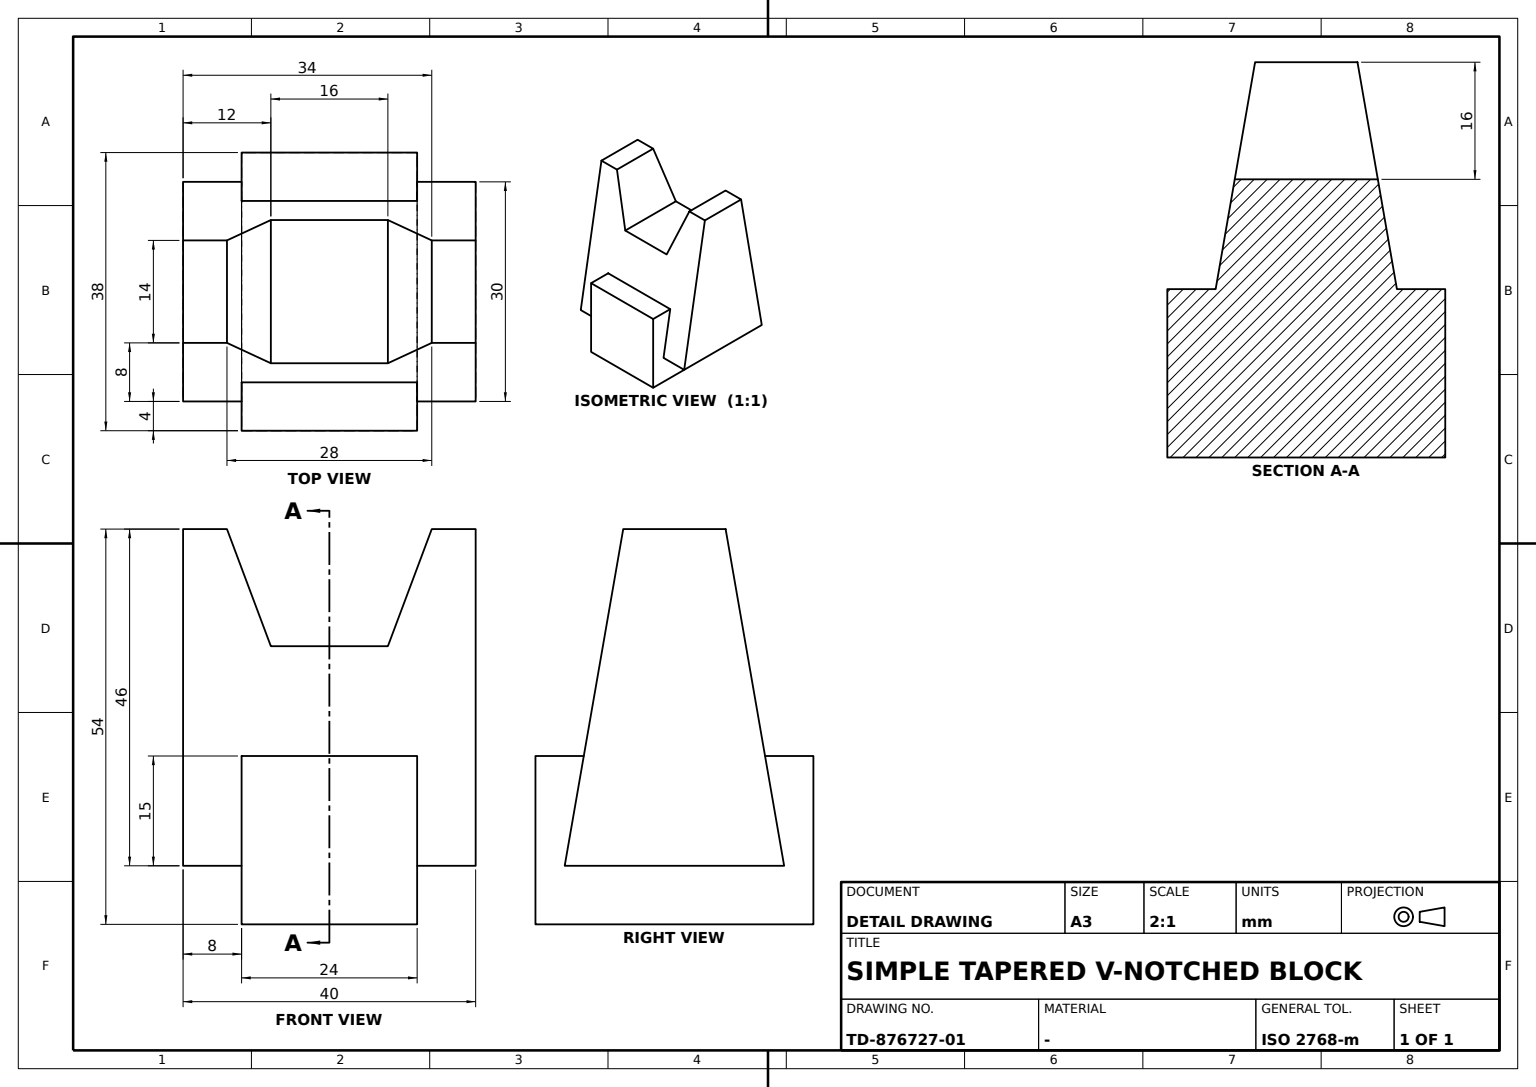
ISO-10303-21;
HEADER;
FILE_DESCRIPTION((''),'2;1');
FILE_NAME('','',(''),(''),'','','');
FILE_SCHEMA(('AUTOMOTIVE_DESIGN'));
ENDSEC;
DATA;
#1=APPLICATION_CONTEXT('');
#2=PRODUCT_CONTEXT('',#1,'mechanical');
#3=PRODUCT('','','',(#2));
#4=PRODUCT_DEFINITION_FORMATION('','',#3);
#5=PRODUCT_DEFINITION_CONTEXT('',#1,'design');
#6=PRODUCT_DEFINITION('','',#4,#5);
#7=PRODUCT_DEFINITION_SHAPE('','',#6);
#8=(LENGTH_UNIT()NAMED_UNIT(*)SI_UNIT(.MILLI.,.METRE.));
#9=(NAMED_UNIT(*)PLANE_ANGLE_UNIT()SI_UNIT($,.RADIAN.));
#10=(NAMED_UNIT(*)SI_UNIT($,.STERADIAN.)SOLID_ANGLE_UNIT());
#11=UNCERTAINTY_MEASURE_WITH_UNIT(LENGTH_MEASURE(0.005),#8,'distance_accuracy_value','');
#12=(GEOMETRIC_REPRESENTATION_CONTEXT(3)GLOBAL_UNCERTAINTY_ASSIGNED_CONTEXT((#11))GLOBAL_UNIT_ASSIGNED_CONTEXT((#8,#9,#10))REPRESENTATION_CONTEXT('',''));
#13=CARTESIAN_POINT('',(-7.,14.,46.));
#14=VERTEX_POINT('',#13);
#15=CARTESIAN_POINT('',(7.,14.,46.));
#16=VERTEX_POINT('',#15);
#17=CARTESIAN_POINT('',(0.,14.,46.));
#18=DIRECTION('',(1.,0.,0.));
#19=VECTOR('',#18,1000.);
#20=LINE('',#17,#19);
#21=EDGE_CURVE('',#14,#16,#20,.T.);
#22=ORIENTED_EDGE('',*,*,#21,.F.);
#23=CARTESIAN_POINT('',(-9.782609,8.,30.));
#24=VERTEX_POINT('',#23);
#25=CARTESIAN_POINT('',(-9.529906,8.54489,31.453041));
#26=DIRECTION('',(-0.160722869,-0.346558687,-0.924156499));
#27=VECTOR('',#26,1000.);
#28=LINE('',#25,#27);
#29=EDGE_CURVE('',#14,#24,#28,.T.);
#30=ORIENTED_EDGE('',*,*,#29,.T.);
#31=CARTESIAN_POINT('',(9.782609,8.,30.));
#32=VERTEX_POINT('',#31);
#33=CARTESIAN_POINT('',(0.,8.,30.));
#34=LINE('',#33,#19);
#35=EDGE_CURVE('',#24,#32,#34,.T.);
#36=ORIENTED_EDGE('',*,*,#35,.T.);
#37=CARTESIAN_POINT('',(9.529906,8.54489,31.453041));
#38=DIRECTION('',(0.160722869,-0.346558687,-0.924156499));
#39=VECTOR('',#38,1000.);
#40=LINE('',#37,#39);
#41=EDGE_CURVE('',#16,#32,#40,.T.);
#42=ORIENTED_EDGE('',*,*,#41,.F.);
#43=EDGE_LOOP('',(#22,#30,#36,#42));
#44=FACE_BOUND('',#43,.T.);
#45=DIRECTION('',(0.,0.936329178,-0.351123442));
#46=DIRECTION('',(0.,0.351123442,0.936329178));
#47=AXIS2_PLACEMENT_3D('',#33,#45,#46);
#48=PLANE('',#47);
#49=ADVANCED_FACE('',(#44),#48,.F.);
#50=CARTESIAN_POINT('',(-15.,-20.,0.));
#51=VERTEX_POINT('',#50);
#52=CARTESIAN_POINT('',(15.,-20.,0.));
#53=VERTEX_POINT('',#52);
#54=CARTESIAN_POINT('',(0.,-20.,0.));
#55=LINE('',#54,#19);
#56=EDGE_CURVE('',#51,#53,#55,.T.);
#57=ORIENTED_EDGE('',*,*,#56,.T.);
#58=CARTESIAN_POINT('',(7.,-20.,46.));
#59=VERTEX_POINT('',#58);
#60=DIRECTION('',(-0.171341175,0.,0.985211755));
#61=VECTOR('',#60,1000.);
#62=LINE('',#52,#61);
#63=EDGE_CURVE('',#53,#59,#62,.T.);
#64=ORIENTED_EDGE('',*,*,#63,.T.);
#65=CARTESIAN_POINT('',(-7.,-20.,46.));
#66=VERTEX_POINT('',#65);
#67=CARTESIAN_POINT('',(0.,-20.,46.));
#68=LINE('',#67,#19);
#69=EDGE_CURVE('',#66,#59,#68,.T.);
#70=ORIENTED_EDGE('',*,*,#69,.F.);
#71=DIRECTION('',(0.171341175,0.,0.985211755));
#72=VECTOR('',#71,1000.);
#73=LINE('',#50,#72);
#74=EDGE_CURVE('',#51,#66,#73,.T.);
#75=ORIENTED_EDGE('',*,*,#74,.F.);
#76=EDGE_LOOP('',(#57,#64,#70,#75));
#77=FACE_BOUND('',#76,.T.);
#78=DIRECTION('',(0.,1.,0.));
#79=DIRECTION('',(0.,0.,1.));
#80=AXIS2_PLACEMENT_3D('',#54,#78,#79);
#81=PLANE('',#80);
#82=ADVANCED_FACE('',(#77),#81,.F.);
#83=CARTESIAN_POINT('',(7.,-14.,46.));
#84=VERTEX_POINT('',#83);
#85=CARTESIAN_POINT('',(9.782609,-8.,30.));
#86=VERTEX_POINT('',#85);
#87=CARTESIAN_POINT('',(14.818975,2.859665,1.040892));
#88=DIRECTION('',(0.160722869,0.346558687,-0.924156499));
#89=VECTOR('',#88,1000.);
#90=LINE('',#87,#89);
#91=EDGE_CURVE('',#84,#86,#90,.T.);
#92=ORIENTED_EDGE('',*,*,#91,.T.);
#93=CARTESIAN_POINT('',(-9.782609,-8.,30.));
#94=VERTEX_POINT('',#93);
#95=CARTESIAN_POINT('',(0.,-8.,30.));
#96=LINE('',#95,#19);
#97=EDGE_CURVE('',#94,#86,#96,.T.);
#98=ORIENTED_EDGE('',*,*,#97,.F.);
#99=CARTESIAN_POINT('',(-7.,-14.,46.));
#100=VERTEX_POINT('',#99);
#101=CARTESIAN_POINT('',(-14.818975,2.859665,1.040892));
#102=DIRECTION('',(-0.160722869,0.346558687,-0.924156499));
#103=VECTOR('',#102,1000.);
#104=LINE('',#101,#103);
#105=EDGE_CURVE('',#100,#94,#104,.T.);
#106=ORIENTED_EDGE('',*,*,#105,.F.);
#107=CARTESIAN_POINT('',(0.,-14.,46.));
#108=LINE('',#107,#19);
#109=EDGE_CURVE('',#100,#84,#108,.T.);
#110=ORIENTED_EDGE('',*,*,#109,.T.);
#111=EDGE_LOOP('',(#92,#98,#106,#110));
#112=FACE_BOUND('',#111,.T.);
#113=DIRECTION('',(0.,-0.936329178,-0.351123442));
#114=DIRECTION('',(0.,0.351123442,-0.936329178));
#115=AXIS2_PLACEMENT_3D('',#107,#113,#114);
#116=PLANE('',#115);
#117=ADVANCED_FACE('',(#112),#116,.F.);
#118=CARTESIAN_POINT('',(19.,-12.,15.));
#119=VERTEX_POINT('',#118);
#120=CARTESIAN_POINT('',(19.,12.,15.));
#121=VERTEX_POINT('',#120);
#122=CARTESIAN_POINT('',(19.,0.,15.));
#123=VECTOR('',#78,1000.);
#124=LINE('',#122,#123);
#125=EDGE_CURVE('',#119,#121,#124,.T.);
#126=ORIENTED_EDGE('',*,*,#125,.F.);
#127=CARTESIAN_POINT('',(19.,-12.,-8.));
#128=VERTEX_POINT('',#127);
#129=CARTESIAN_POINT('',(19.,-12.,0.));
#130=DIRECTION('',(0.,0.,-1.));
#131=VECTOR('',#130,1000.);
#132=LINE('',#129,#131);
#133=EDGE_CURVE('',#119,#128,#132,.T.);
#134=ORIENTED_EDGE('',*,*,#133,.T.);
#135=CARTESIAN_POINT('',(19.,12.,-8.));
#136=VERTEX_POINT('',#135);
#137=CARTESIAN_POINT('',(19.,0.,-8.));
#138=DIRECTION('',(0.,-1.,0.));
#139=VECTOR('',#138,1000.);
#140=LINE('',#137,#139);
#141=EDGE_CURVE('',#136,#128,#140,.T.);
#142=ORIENTED_EDGE('',*,*,#141,.F.);
#143=VECTOR('',#79,1000.);
#144=LINE('',#120,#143);
#145=EDGE_CURVE('',#136,#121,#144,.T.);
#146=ORIENTED_EDGE('',*,*,#145,.T.);
#147=EDGE_LOOP('',(#126,#134,#142,#146));
#148=FACE_BOUND('',#147,.T.);
#149=CARTESIAN_POINT('',(19.,0.,0.));
#150=AXIS2_PLACEMENT_3D('',#149,#18,#78);
#151=PLANE('',#150);
#152=ADVANCED_FACE('',(#148),#151,.T.);
#153=CARTESIAN_POINT('',(-7.,20.,46.));
#154=VERTEX_POINT('',#153);
#155=LINE('',#13,#139);
#156=EDGE_CURVE('',#154,#14,#155,.T.);
#157=ORIENTED_EDGE('',*,*,#156,.F.);
#158=CARTESIAN_POINT('',(-15.,20.,0.));
#159=VERTEX_POINT('',#158);
#160=CARTESIAN_POINT('',(-6.794495,20.,47.181651));
#161=LINE('',#160,#72);
#162=EDGE_CURVE('',#159,#154,#161,.T.);
#163=ORIENTED_EDGE('',*,*,#162,.F.);
#164=CARTESIAN_POINT('',(-15.,12.,0.));
#165=VERTEX_POINT('',#164);
#166=CARTESIAN_POINT('',(-15.,0.,0.));
#167=LINE('',#166,#139);
#168=EDGE_CURVE('',#159,#165,#167,.T.);
#169=ORIENTED_EDGE('',*,*,#168,.T.);
#170=CARTESIAN_POINT('',(-12.391304,12.,15.));
#171=VERTEX_POINT('',#170);
#172=CARTESIAN_POINT('',(-12.027523,12.,17.091743));
#173=LINE('',#172,#72);
#174=EDGE_CURVE('',#165,#171,#173,.T.);
#175=ORIENTED_EDGE('',*,*,#174,.T.);
#176=CARTESIAN_POINT('',(-12.391304,-12.,15.));
#177=VERTEX_POINT('',#176);
#178=CARTESIAN_POINT('',(-12.391304,0.,15.));
#179=LINE('',#178,#123);
#180=EDGE_CURVE('',#177,#171,#179,.T.);
#181=ORIENTED_EDGE('',*,*,#180,.F.);
#182=CARTESIAN_POINT('',(-15.,-12.,0.));
#183=VERTEX_POINT('',#182);
#184=CARTESIAN_POINT('',(-12.027523,-12.,17.091743));
#185=LINE('',#184,#72);
#186=EDGE_CURVE('',#183,#177,#185,.T.);
#187=ORIENTED_EDGE('',*,*,#186,.F.);
#188=EDGE_CURVE('',#183,#51,#167,.T.);
#189=ORIENTED_EDGE('',*,*,#188,.T.);
#190=ORIENTED_EDGE('',*,*,#74,.T.);
#191=EDGE_CURVE('',#100,#66,#155,.T.);
#192=ORIENTED_EDGE('',*,*,#191,.F.);
#193=ORIENTED_EDGE('',*,*,#105,.T.);
#194=CARTESIAN_POINT('',(-9.782609,0.,30.));
#195=LINE('',#194,#123);
#196=EDGE_CURVE('',#94,#24,#195,.T.);
#197=ORIENTED_EDGE('',*,*,#196,.T.);
#198=ORIENTED_EDGE('',*,*,#29,.F.);
#199=EDGE_LOOP('',(#157,#163,#169,#175,#181,#187,#189,#190,#192,#193,#197,#198));
#200=FACE_BOUND('',#199,.T.);
#201=DIRECTION('',(0.985211755,0.,-0.171341175));
#202=AXIS2_PLACEMENT_3D('',#166,#201,#71);
#203=PLANE('',#202);
#204=ADVANCED_FACE('',(#200),#203,.F.);
#205=CARTESIAN_POINT('',(7.,20.,46.));
#206=VERTEX_POINT('',#205);
#207=CARTESIAN_POINT('',(0.,20.,46.));
#208=LINE('',#207,#19);
#209=EDGE_CURVE('',#154,#206,#208,.T.);
#210=ORIENTED_EDGE('',*,*,#209,.T.);
#211=CARTESIAN_POINT('',(15.,20.,0.));
#212=VERTEX_POINT('',#211);
#213=CARTESIAN_POINT('',(6.794495,20.,47.181651));
#214=LINE('',#213,#61);
#215=EDGE_CURVE('',#212,#206,#214,.T.);
#216=ORIENTED_EDGE('',*,*,#215,.F.);
#217=CARTESIAN_POINT('',(0.,20.,0.));
#218=LINE('',#217,#19);
#219=EDGE_CURVE('',#159,#212,#218,.T.);
#220=ORIENTED_EDGE('',*,*,#219,.F.);
#221=ORIENTED_EDGE('',*,*,#162,.T.);
#222=EDGE_LOOP('',(#210,#216,#220,#221));
#223=FACE_BOUND('',#222,.T.);
#224=AXIS2_PLACEMENT_3D('',#207,#138,#130);
#225=PLANE('',#224);
#226=ADVANCED_FACE('',(#223),#225,.F.);
#227=CARTESIAN_POINT('',(-19.,-12.,-8.));
#228=VERTEX_POINT('',#227);
#229=CARTESIAN_POINT('',(0.,-12.,-8.));
#230=LINE('',#229,#19);
#231=EDGE_CURVE('',#228,#128,#230,.T.);
#232=ORIENTED_EDGE('',*,*,#231,.T.);
#233=ORIENTED_EDGE('',*,*,#133,.F.);
#234=CARTESIAN_POINT('',(12.391304,-12.,15.));
#235=VERTEX_POINT('',#234);
#236=CARTESIAN_POINT('',(0.,-12.,15.));
#237=LINE('',#236,#19);
#238=EDGE_CURVE('',#235,#119,#237,.T.);
#239=ORIENTED_EDGE('',*,*,#238,.F.);
#240=CARTESIAN_POINT('',(15.,-12.,0.));
#241=VERTEX_POINT('',#240);
#242=CARTESIAN_POINT('',(12.027523,-12.,17.091743));
#243=LINE('',#242,#61);
#244=EDGE_CURVE('',#241,#235,#243,.T.);
#245=ORIENTED_EDGE('',*,*,#244,.F.);
#246=CARTESIAN_POINT('',(0.,-12.,0.));
#247=LINE('',#246,#19);
#248=EDGE_CURVE('',#183,#241,#247,.T.);
#249=ORIENTED_EDGE('',*,*,#248,.F.);
#250=ORIENTED_EDGE('',*,*,#186,.T.);
#251=CARTESIAN_POINT('',(-19.,-12.,15.));
#252=VERTEX_POINT('',#251);
#253=EDGE_CURVE('',#252,#177,#237,.T.);
#254=ORIENTED_EDGE('',*,*,#253,.F.);
#255=CARTESIAN_POINT('',(-19.,-12.,0.));
#256=LINE('',#255,#131);
#257=EDGE_CURVE('',#252,#228,#256,.T.);
#258=ORIENTED_EDGE('',*,*,#257,.T.);
#259=EDGE_LOOP('',(#232,#233,#239,#245,#249,#250,#254,#258));
#260=FACE_BOUND('',#259,.T.);
#261=AXIS2_PLACEMENT_3D('',#236,#138,#130);
#262=PLANE('',#261);
#263=ADVANCED_FACE('',(#260),#262,.T.);
#264=CARTESIAN_POINT('',(9.782609,0.,30.));
#265=LINE('',#264,#123);
#266=EDGE_CURVE('',#86,#32,#265,.T.);
#267=ORIENTED_EDGE('',*,*,#266,.T.);
#268=ORIENTED_EDGE('',*,*,#35,.F.);
#269=ORIENTED_EDGE('',*,*,#196,.F.);
#270=ORIENTED_EDGE('',*,*,#97,.T.);
#271=EDGE_LOOP('',(#267,#268,#269,#270));
#272=FACE_BOUND('',#271,.T.);
#273=AXIS2_PLACEMENT_3D('',#95,#130,#78);
#274=PLANE('',#273);
#275=ADVANCED_FACE('',(#272),#274,.F.);
#276=ORIENTED_EDGE('',*,*,#191,.T.);
#277=ORIENTED_EDGE('',*,*,#69,.T.);
#278=LINE('',#15,#139);
#279=EDGE_CURVE('',#84,#59,#278,.T.);
#280=ORIENTED_EDGE('',*,*,#279,.F.);
#281=ORIENTED_EDGE('',*,*,#109,.F.);
#282=EDGE_LOOP('',(#276,#277,#280,#281));
#283=FACE_BOUND('',#282,.T.);
#284=AXIS2_PLACEMENT_3D('',#17,#130,#78);
#285=PLANE('',#284);
#286=ADVANCED_FACE('',(#283),#285,.F.);
#287=ORIENTED_EDGE('',*,*,#141,.T.);
#288=ORIENTED_EDGE('',*,*,#231,.F.);
#289=CARTESIAN_POINT('',(-19.,12.,-8.));
#290=VERTEX_POINT('',#289);
#291=CARTESIAN_POINT('',(-19.,0.,-8.));
#292=LINE('',#291,#139);
#293=EDGE_CURVE('',#290,#228,#292,.T.);
#294=ORIENTED_EDGE('',*,*,#293,.F.);
#295=CARTESIAN_POINT('',(0.,12.,-8.));
#296=LINE('',#295,#19);
#297=EDGE_CURVE('',#290,#136,#296,.T.);
#298=ORIENTED_EDGE('',*,*,#297,.T.);
#299=EDGE_LOOP('',(#287,#288,#294,#298));
#300=FACE_BOUND('',#299,.T.);
#301=AXIS2_PLACEMENT_3D('',#295,#79,#138);
#302=PLANE('',#301);
#303=ADVANCED_FACE('',(#300),#302,.F.);
#304=CARTESIAN_POINT('',(15.,12.,0.));
#305=VERTEX_POINT('',#304);
#306=CARTESIAN_POINT('',(15.,0.,0.));
#307=LINE('',#306,#139);
#308=EDGE_CURVE('',#212,#305,#307,.T.);
#309=ORIENTED_EDGE('',*,*,#308,.F.);
#310=ORIENTED_EDGE('',*,*,#215,.T.);
#311=EDGE_CURVE('',#206,#16,#278,.T.);
#312=ORIENTED_EDGE('',*,*,#311,.T.);
#313=ORIENTED_EDGE('',*,*,#41,.T.);
#314=ORIENTED_EDGE('',*,*,#266,.F.);
#315=ORIENTED_EDGE('',*,*,#91,.F.);
#316=ORIENTED_EDGE('',*,*,#279,.T.);
#317=ORIENTED_EDGE('',*,*,#63,.F.);
#318=EDGE_CURVE('',#241,#53,#307,.T.);
#319=ORIENTED_EDGE('',*,*,#318,.F.);
#320=ORIENTED_EDGE('',*,*,#244,.T.);
#321=CARTESIAN_POINT('',(12.391304,12.,15.));
#322=VERTEX_POINT('',#321);
#323=CARTESIAN_POINT('',(12.391304,0.,15.));
#324=LINE('',#323,#123);
#325=EDGE_CURVE('',#235,#322,#324,.T.);
#326=ORIENTED_EDGE('',*,*,#325,.T.);
#327=CARTESIAN_POINT('',(12.027523,12.,17.091743));
#328=LINE('',#327,#61);
#329=EDGE_CURVE('',#305,#322,#328,.T.);
#330=ORIENTED_EDGE('',*,*,#329,.F.);
#331=EDGE_LOOP('',(#309,#310,#312,#313,#314,#315,#316,#317,#319,#320,#326,#330));
#332=FACE_BOUND('',#331,.T.);
#333=DIRECTION('',(0.985211755,0.,0.171341175));
#334=AXIS2_PLACEMENT_3D('',#306,#333,#60);
#335=PLANE('',#334);
#336=ADVANCED_FACE('',(#332),#335,.T.);
#337=ORIENTED_EDGE('',*,*,#257,.F.);
#338=CARTESIAN_POINT('',(-19.,12.,15.));
#339=VERTEX_POINT('',#338);
#340=CARTESIAN_POINT('',(-19.,0.,15.));
#341=LINE('',#340,#123);
#342=EDGE_CURVE('',#252,#339,#341,.T.);
#343=ORIENTED_EDGE('',*,*,#342,.T.);
#344=LINE('',#338,#143);
#345=EDGE_CURVE('',#290,#339,#344,.T.);
#346=ORIENTED_EDGE('',*,*,#345,.F.);
#347=ORIENTED_EDGE('',*,*,#293,.T.);
#348=EDGE_LOOP('',(#337,#343,#346,#347));
#349=FACE_BOUND('',#348,.T.);
#350=CARTESIAN_POINT('',(-19.,0.,0.));
#351=AXIS2_PLACEMENT_3D('',#350,#18,#78);
#352=PLANE('',#351);
#353=ADVANCED_FACE('',(#349),#352,.F.);
#354=CARTESIAN_POINT('',(0.,12.,15.));
#355=LINE('',#354,#19);
#356=EDGE_CURVE('',#339,#171,#355,.T.);
#357=ORIENTED_EDGE('',*,*,#356,.F.);
#358=ORIENTED_EDGE('',*,*,#342,.F.);
#359=ORIENTED_EDGE('',*,*,#253,.T.);
#360=ORIENTED_EDGE('',*,*,#180,.T.);
#361=EDGE_LOOP('',(#357,#358,#359,#360));
#362=FACE_BOUND('',#361,.T.);
#363=AXIS2_PLACEMENT_3D('',#236,#130,#78);
#364=PLANE('',#363);
#365=ADVANCED_FACE('',(#362),#364,.F.);
#366=ORIENTED_EDGE('',*,*,#238,.T.);
#367=ORIENTED_EDGE('',*,*,#125,.T.);
#368=EDGE_CURVE('',#322,#121,#355,.T.);
#369=ORIENTED_EDGE('',*,*,#368,.F.);
#370=ORIENTED_EDGE('',*,*,#325,.F.);
#371=EDGE_LOOP('',(#366,#367,#369,#370));
#372=FACE_BOUND('',#371,.T.);
#373=ADVANCED_FACE('',(#372),#364,.F.);
#374=ORIENTED_EDGE('',*,*,#21,.T.);
#375=ORIENTED_EDGE('',*,*,#311,.F.);
#376=ORIENTED_EDGE('',*,*,#209,.F.);
#377=ORIENTED_EDGE('',*,*,#156,.T.);
#378=EDGE_LOOP('',(#374,#375,#376,#377));
#379=FACE_BOUND('',#378,.T.);
#380=ADVANCED_FACE('',(#379),#285,.F.);
#381=ORIENTED_EDGE('',*,*,#308,.T.);
#382=CARTESIAN_POINT('',(0.,12.,0.));
#383=LINE('',#382,#19);
#384=EDGE_CURVE('',#165,#305,#383,.T.);
#385=ORIENTED_EDGE('',*,*,#384,.F.);
#386=ORIENTED_EDGE('',*,*,#168,.F.);
#387=ORIENTED_EDGE('',*,*,#219,.T.);
#388=EDGE_LOOP('',(#381,#385,#386,#387));
#389=FACE_BOUND('',#388,.T.);
#390=CARTESIAN_POINT('',(0.,14.,0.));
#391=AXIS2_PLACEMENT_3D('',#390,#79,#138);
#392=PLANE('',#391);
#393=ADVANCED_FACE('',(#389),#392,.F.);
#394=ORIENTED_EDGE('',*,*,#145,.F.);
#395=ORIENTED_EDGE('',*,*,#297,.F.);
#396=ORIENTED_EDGE('',*,*,#345,.T.);
#397=ORIENTED_EDGE('',*,*,#356,.T.);
#398=ORIENTED_EDGE('',*,*,#174,.F.);
#399=ORIENTED_EDGE('',*,*,#384,.T.);
#400=ORIENTED_EDGE('',*,*,#329,.T.);
#401=ORIENTED_EDGE('',*,*,#368,.T.);
#402=EDGE_LOOP('',(#394,#395,#396,#397,#398,#399,#400,#401));
#403=FACE_BOUND('',#402,.T.);
#404=AXIS2_PLACEMENT_3D('',#354,#138,#130);
#405=PLANE('',#404);
#406=ADVANCED_FACE('',(#403),#405,.F.);
#407=ORIENTED_EDGE('',*,*,#56,.F.);
#408=ORIENTED_EDGE('',*,*,#188,.F.);
#409=ORIENTED_EDGE('',*,*,#248,.T.);
#410=ORIENTED_EDGE('',*,*,#318,.T.);
#411=EDGE_LOOP('',(#407,#408,#409,#410));
#412=FACE_BOUND('',#411,.T.);
#413=ADVANCED_FACE('',(#412),#392,.F.);
#414=CLOSED_SHELL('',(#49,#82,#117,#152,#204,#226,#263,#275,#286,#303,#336,#353,#365,#373,#380,#393,#406,#413));
#415=MANIFOLD_SOLID_BREP('',#414);
#416=ADVANCED_BREP_SHAPE_REPRESENTATION('',(#415),#12);
#417=SHAPE_DEFINITION_REPRESENTATION(#7,#416);
ENDSEC;
END-ISO-10303-21;
